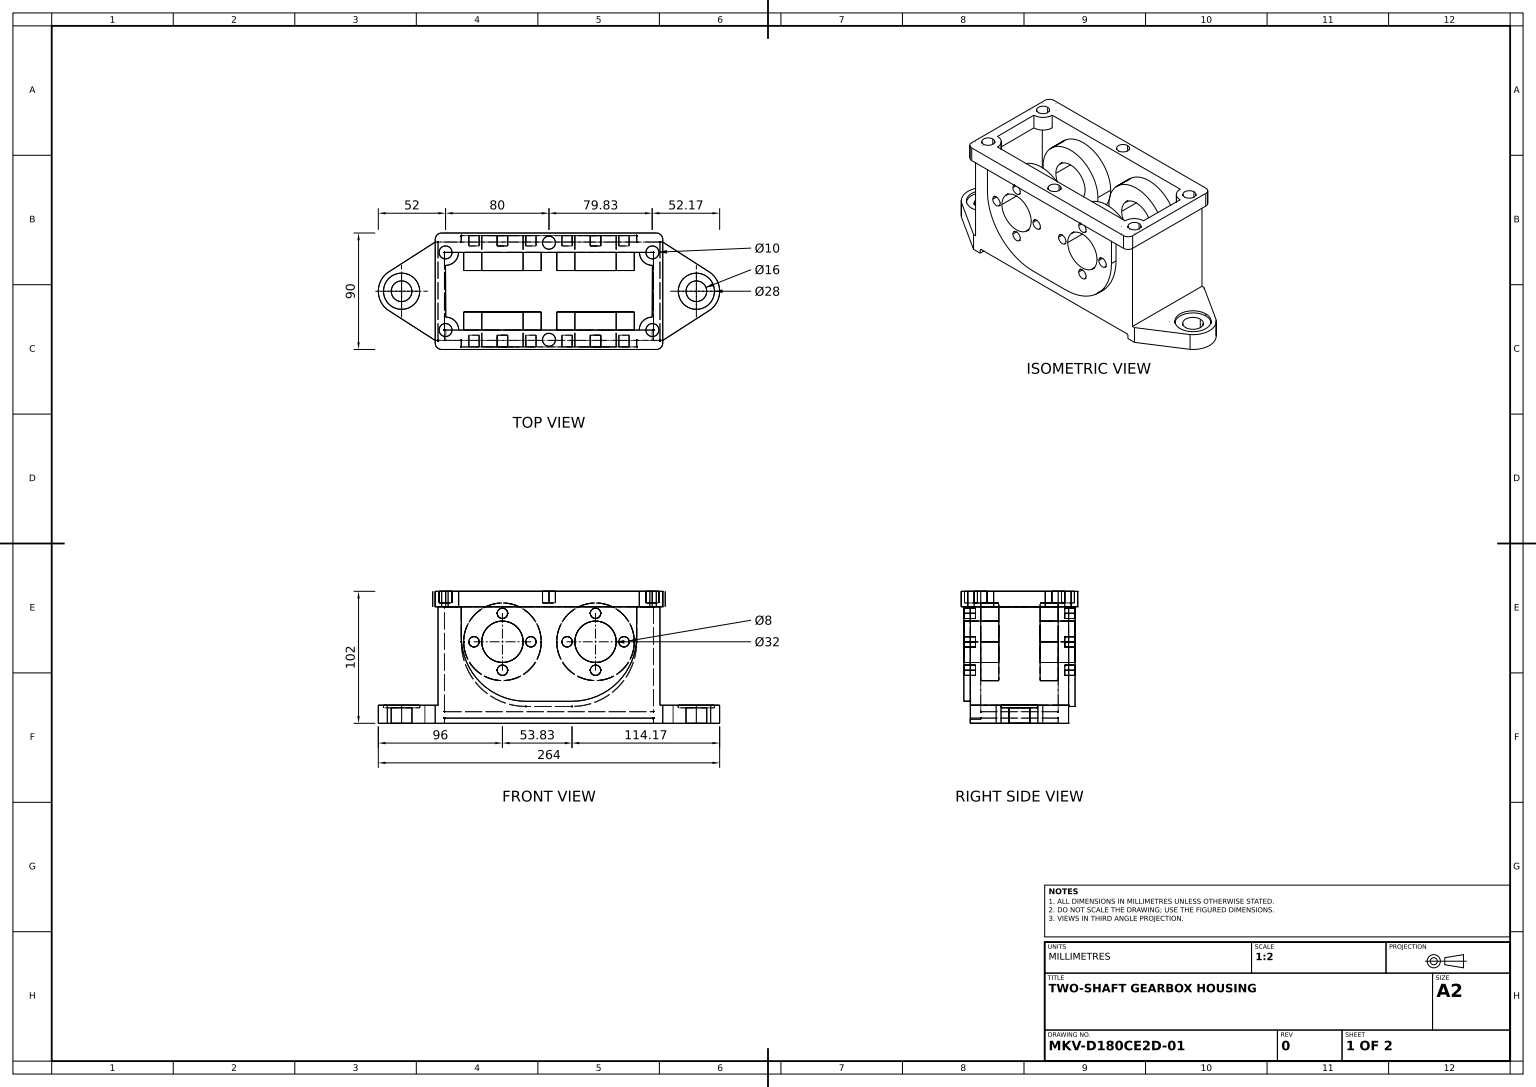
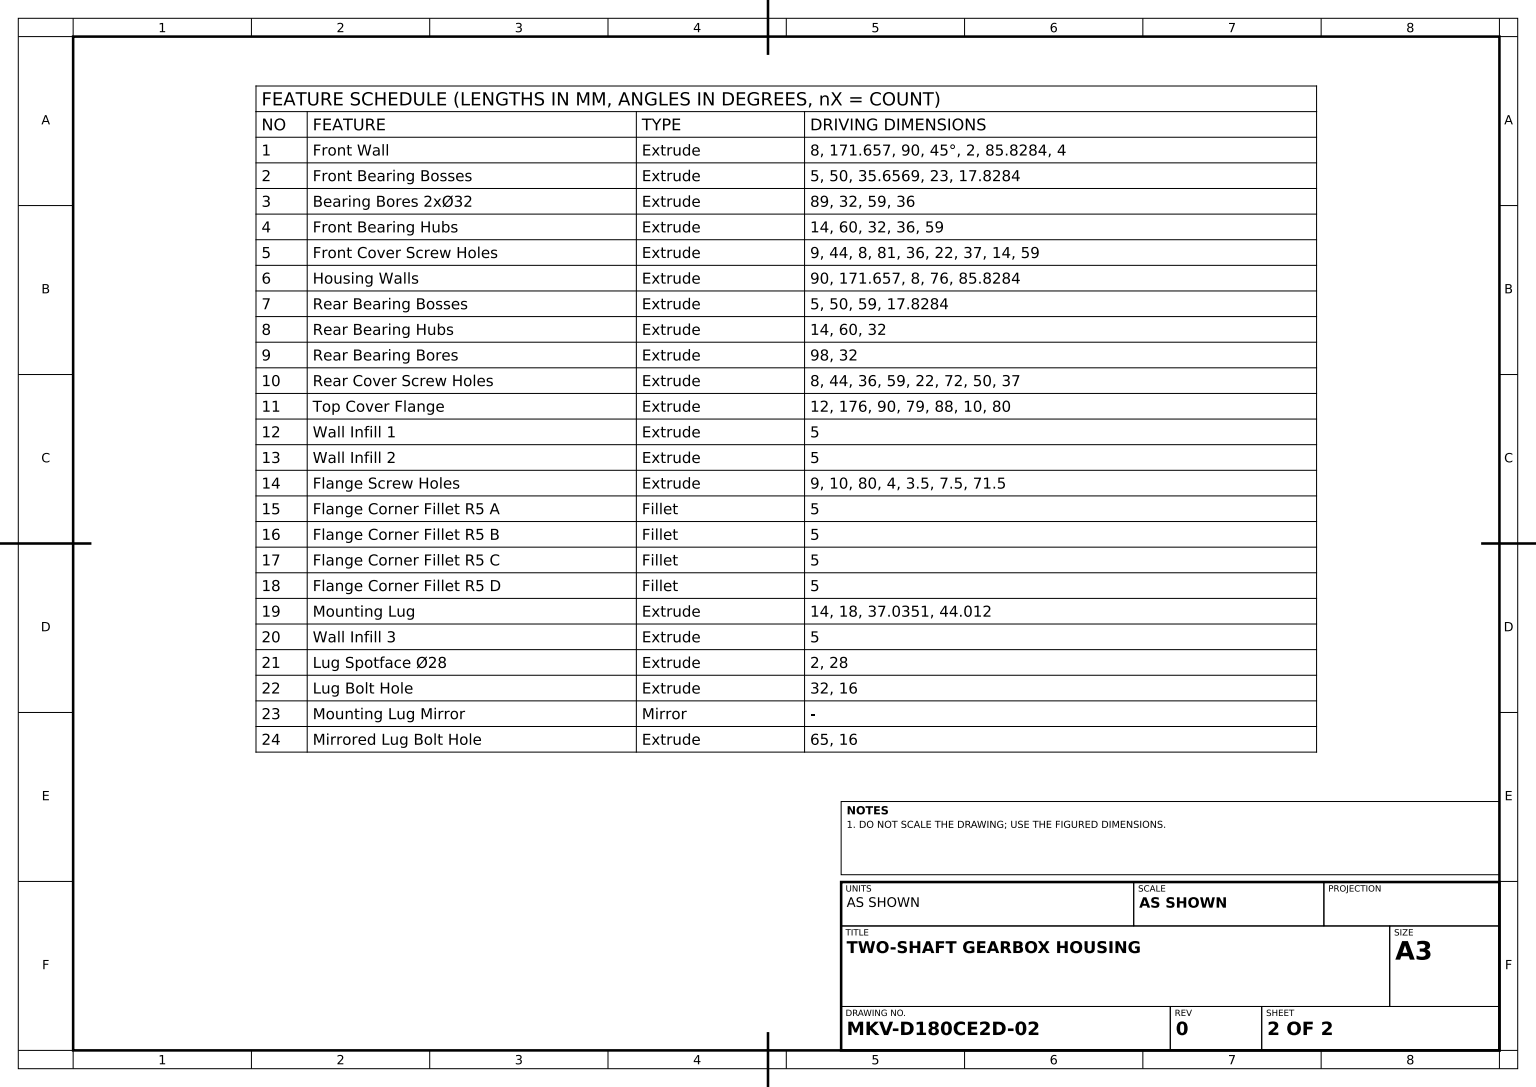
solid
v1 (-80,89,-59)
v2 (-80,98,-59)
e1 v1 v2 LINE
v3 (-80,98,-69)
e2 v2 v3 CIRCLE(AX(P(-80,98,-64),D(0,1,0),D(0,0,1)),5)
v4 (-80,89,-69)
e3 v4 v3 LINE
e4 v1 v4 CIRCLE(AX(P(-80,89,-64),D(0,1,0),D(0,0,1)),5)
face CYL(AX(P(-80,89,-64),D(0,1,0),D(0,0,1)),5) rev [e1 e2 -e3 -e4]
v5 (40,81,-77)
v6 (32,81,-77)
e5 v5 v6 CIRCLE(AX(P(36,81,-77),D(0,0,-1),D(1,0,0)),4)
v7 (32,81,-69)
e6 v7 v6 LINE
v8 (40,81,-69)
e7 v8 v7 CIRCLE(AX(P(36,81,-69),D(0,0,-1),D(1,0,0)),4)
e8 v8 v5 LINE
face CYL(AX(P(36,81,-69),D(0,0,-1),D(-1,0,0)),4) rev [e5 -e6 -e7 e8]
v9 (-69.828427,98,-4)
v10 (-79.828427,98,-14)
e9 v9 v10 CIRCLE(AX(P(-79.828427,98,-4),D(0,1,0),D(0,0,1)),10)
v11 (-69.828427,86,-4)
e10 v9 v11 LINE
v12 (-79.828427,86,-14)
e11 v11 v12 CIRCLE(AX(P(-79.828427,86,-4),D(0,1,0),D(0,0,1)),10)
e12 v10 v12 LINE
face CYL(AX(P(-79.828427,98,-4),D(0,-1,0),D(0,0,-1)),10) [-e9 e10 e11 -e12]
v13 (80,98,-59)
v14 (80,98,-69)
e13 v13 v14 CIRCLE(AX(P(80,98,-64),D(0,1,0),D(0,0,1)),5)
e14 v14 v13 CIRCLE(AX(P(80,98,-64),D(0,1,0),D(0,0,1)),5)
v15 (80,98,1)
v16 (80,98,-9)
e15 v15 v16 CIRCLE(AX(P(80,98,-4),D(0,1,0),D(0,0,-1)),5)
e16 v16 v15 CIRCLE(AX(P(80,98,-4),D(0,1,0),D(0,0,-1)),5)
v17 (0,98,-66.5)
v18 (0,98,-76.5)
e17 v17 v18 CIRCLE(AX(P(0,98,-71.5),D(0,1,0),D(0,0,1)),5)
e18 v18 v17 CIRCLE(AX(P(0,98,-71.5),D(0,1,0),D(0,0,1)),5)
v19 (83,98,-79)
v20 (-83,98,-79)
e19 v19 v20 LINE
v21 (-88,98,-74)
e20 v20 v21 CIRCLE(AX(P(-83,98,-74),D(0,1,0),D(0,0,1)),5)
v22 (-88,98,6)
e21 v21 v22 LINE
v23 (-83,98,11)
e22 v22 v23 CIRCLE(AX(P(-83,98,6),D(0,1,0),D(0,0,1)),5)
v24 (83,98,11)
e23 v23 v24 LINE
v25 (88,98,6)
e24 v24 v25 CIRCLE(AX(P(83,98,6),D(0,1,0),D(0,0,1)),5)
v26 (88,98,-74)
e25 v25 v26 LINE
e26 v26 v19 CIRCLE(AX(P(83,98,-74),D(0,1,0),D(0,0,1)),5)
e27 v3 v2 CIRCLE(AX(P(-80,98,-64),D(0,1,0),D(0,0,1)),5)
v27 (0,98,-1.5)
v28 (0,98,8.5)
e28 v27 v28 CIRCLE(AX(P(0,98,3.5),D(0,1,0),D(0,0,-1)),5)
e29 v28 v27 CIRCLE(AX(P(0,98,3.5),D(0,1,0),D(0,0,-1)),5)
v29 (-80,98,1)
v30 (-80,98,-9)
e30 v29 v30 CIRCLE(AX(P(-80,98,-4),D(0,1,0),D(0,0,-1)),5)
e31 v30 v29 CIRCLE(AX(P(-80,98,-4),D(0,1,0),D(0,0,-1)),5)
v31 (69.828427,98,-4)
v32 (79.828427,98,-14)
e32 v31 v32 CIRCLE(AX(P(79.828427,98,-4),D(0,-1,0),D(0,0,1)),10)
e33 v31 v9 LINE
v33 (-80,98,-54)
e34 v10 v33 LINE
v34 (-70,98,-64)
e35 v33 v34 CIRCLE(AX(P(-80,98,-64),D(0,1,0),D(0,0,1)),10)
v35 (70,98,-64)
e36 v34 v35 LINE
v36 (80,98,-54)
e37 v36 v35 CIRCLE(AX(P(80,98,-64),D(0,-1,0),D(0,0,1)),10)
e38 v36 v32 LINE
face PLANE(AX(P(0,98,0),D(0,1,0),D(0,0,1))) [-e13 -e14] [-e15 -e16] [-e17 -e18] [e19 e20 e21 e22 e23 e24 e25 e26] [-e27 -e2] [-e28 -e29] [-e30 -e31] [-e32 e33 e9 e34 e35 e36 -e37 e38]
v37 (70,86,-64)
e39 v35 v37 LINE
v38 (80,86,-54)
e40 v38 v37 CIRCLE(AX(P(80,86,-64),D(0,-1,0),D(0,0,1)),10)
e41 v36 v38 LINE
face CYL(AX(P(80,98,-64),D(0,-1,0),D(0,0,-1)),10) [e39 -e40 -e41 e37]
v39 (80,89,1)
e42 v39 v15 LINE
v40 (80,89,-9)
e43 v40 v16 LINE
e44 v39 v40 CIRCLE(AX(P(80,89,-4),D(0,1,0),D(0,0,-1)),5)
face CYL(AX(P(80,89,-4),D(0,1,0),D(0,0,1)),5) rev [e42 e15 -e43 -e44]
v41 (67.828427,59,-72)
v42 (17.828427,9,-72)
e45 v41 v42 CIRCLE(AX(P(17.828427,59,-72),D(0,0,-1),D(-1,0,0)),50)
v43 (17.828427,9,-77)
e46 v43 v42 LINE
v44 (67.828427,59,-77)
e47 v44 v43 CIRCLE(AX(P(17.828427,59,-77),D(0,0,-1),D(-1,0,0)),50)
e48 v44 v41 LINE
face CYL(AX(P(17.828427,59,-77),D(0,0,1),D(1,0,0)),50) [e45 -e46 -e47 e48]
v45 (-40,81,-69)
v46 (-40,81,-77)
e49 v45 v46 LINE
v47 (-32,81,-69)
e50 v47 v45 CIRCLE(AX(P(-36,81,-69),D(0,0,-1),D(-1,0,0)),4)
v48 (-32,81,-77)
e51 v47 v48 LINE
e52 v48 v46 CIRCLE(AX(P(-36,81,-77),D(0,0,-1),D(-1,0,0)),4)
face CYL(AX(P(-36,81,-69),D(0,0,-1),D(-1,0,0)),4) rev [-e49 -e50 e51 e52]
v49 (-80.828427,5,-64)
v50 (-80.828427,86,-64)
e53 v49 v50 LINE
v51 (80.828427,5,-64)
e54 v49 v51 LINE
v52 (80.828427,86,-64)
e55 v52 v51 LINE
e56 v37 v52 LINE
v53 (-70,86,-64)
e57 v34 v53 LINE
e58 v50 v53 LINE
v54 (66,59,-64)
v55 (6,59,-64)
e59 v54 v55 CIRCLE(AX(P(36,59,-64),D(0,0,1),D(1,0,0)),30)
e60 v55 v54 CIRCLE(AX(P(36,59,-64),D(0,0,1),D(1,0,0)),30)
v56 (-66,59,-64)
v57 (-6,59,-64)
e61 v56 v57 CIRCLE(AX(P(-36,59,-64),D(0,0,1),D(1,0,0)),30)
e62 v57 v56 CIRCLE(AX(P(-36,59,-64),D(0,0,1),D(1,0,0)),30)
face PLANE(AX(P(0,98,-64),D(0,0,-1),D(-1,0,0))) rev [-e53 e54 -e55 -e56 -e39 -e36 e57 -e58] [-e59 -e60] [-e61 -e62]
v58 (-17.828427,13,4)
v59 (17.828427,13,4)
e63 v58 v59 LINE
v60 (-67.828427,63,4)
e64 v60 v58 CIRCLE(AX(P(-17.828427,63,4),D(0,0,1),D(1,0,0)),50)
v61 (-67.828427,86,4)
e65 v61 v60 LINE
v62 (-85.828427,86,4)
e66 v61 v62 LINE
v63 (-85.828427,10,4)
e67 v62 v63 LINE
v64 (-88,10,4)
e68 v64 v63 LINE
v65 (-88,-4,4)
e69 v64 v65 LINE
v66 (-80.828427,-4,4)
e70 v65 v66 LINE
v67 (-80.828427,-1,4)
e71 v66 v67 LINE
v68 (-79.828427,0,4)
e72 v67 v68 LINE
v69 (79.828427,0,4)
e73 v68 v69 LINE
v70 (80.828427,-1,4)
e74 v69 v70 LINE
v71 (80.828427,-4,4)
e75 v70 v71 LINE
v72 (88,-4,4)
e76 v71 v72 LINE
v73 (88,10,4)
e77 v73 v72 LINE
v74 (85.828427,10,4)
e78 v73 v74 LINE
v75 (85.828427,86,4)
e79 v74 v75 LINE
v76 (67.828427,86,4)
e80 v75 v76 LINE
v77 (67.828427,63,4)
e81 v77 v76 LINE
e82 v59 v77 CIRCLE(AX(P(17.828427,63,4),D(0,0,1),D(1,0,0)),50)
face PLANE(AX(P(0,0,4),D(0,0,-1),D(-1,0,0))) rev [-e63 -e64 -e65 e66 e67 -e68 e69 e70 e71 e72 e73 e74 e75 e76 -e77 e78 e79 e80 -e81 -e82]
v78 (-40,37,-69)
v79 (-32,37,-69)
e83 v78 v79 CIRCLE(AX(P(-36,37,-69),D(0,0,-1),D(-1,0,0)),4)
e84 v79 v78 CIRCLE(AX(P(-36,37,-69),D(0,0,-1),D(-1,0,0)),4)
face PLANE(AX(P(-36,37,-69),D(0,0,-1),D(-1,0,0))) [e83 e84]
v80 (114,8,-42)
v81 (114,8,-26)
e85 v80 v81 CIRCLE(AX(P(114,8,-34),D(0,1,0),D(0,0,1)),8)
e86 v81 v80 CIRCLE(AX(P(114,8,-34),D(0,1,0),D(0,0,1)),8)
v82 (114,8,-20)
v83 (114,8,-48)
e87 v82 v83 CIRCLE(AX(P(114,8,-34),D(0,1,0),D(0,0,1)),14)
e88 v83 v82 CIRCLE(AX(P(114,8,-34),D(0,1,0),D(0,0,1)),14)
face PLANE(AX(P(114,8,-34),D(0,1,0),D(0,0,1))) [-e85 -e86] [e87 e88]
v84 (-32,37,0)
v85 (-40,37,0)
e89 v84 v85 CIRCLE(AX(P(-36,37,0),D(0,0,1),D(1,0,0)),4)
e90 v85 v84 CIRCLE(AX(P(-36,37,0),D(0,0,1),D(1,0,0)),4)
face PLANE(AX(P(-36,37,0),D(0,0,1),D(1,0,0))) [e89 e90]
v86 (-66,59,-18)
v87 (-6,59,-18)
e91 v86 v87 CIRCLE(AX(P(-36,59,-18),D(0,0,-1),D(-1,0,0)),30)
v88 (-66,59,-4)
e92 v86 v88 LINE
v89 (-6,59,-4)
e93 v88 v89 CIRCLE(AX(P(-36,59,-4),D(0,0,-1),D(-1,0,0)),30)
e94 v87 v89 LINE
face CYL(AX(P(-36,59,-18),D(0,0,1),D(1,0,0)),30) [-e91 e92 e93 -e94]
v90 (-88,86,-74)
e95 v21 v90 LINE
v91 (-88,86,6)
e96 v90 v91 LINE
e97 v91 v22 LINE
face PLANE(AX(P(-88,98,0),D(1,0,0),D(0,0,-1))) rev [e95 e96 e97 -e21]
v92 (-32,37,9)
e98 v84 v92 LINE
v93 (-40,37,9)
e99 v92 v93 CIRCLE(AX(P(-36,37,9),D(0,0,1),D(1,0,0)),4)
e100 v85 v93 LINE
face CYL(AX(P(-36,37,0),D(0,0,1),D(1,0,0)),4) rev [e98 e99 -e100 -e89]
v94 (79.828427,86,-14)
e101 v38 v94 LINE
e102 v32 v94 LINE
face PLANE(AX(P(79.766909,98,0.342146),D(0.999990801,0,0.004289282),D(0.004289282,0,-0.999990801))) rev [-e38 e41 e101 -e102]
v95 (-83,86,11)
v96 (83,86,11)
e103 v95 v96 LINE
e104 v96 v24 LINE
e105 v23 v95 LINE
face PLANE(AX(P(0,98,11),D(0,0,-1),D(-1,0,0))) rev [e103 e104 -e23 e105]
v97 (-40,81,9)
v98 (-32,81,9)
e106 v97 v98 CIRCLE(AX(P(-36,81,9),D(0,0,1),D(1,0,0)),4)
v99 (-32,81,0)
e107 v99 v98 LINE
v100 (-40,81,0)
e108 v100 v99 CIRCLE(AX(P(-36,81,0),D(0,0,1),D(1,0,0)),4)
e109 v100 v97 LINE
face CYL(AX(P(-36,81,0),D(0,0,1),D(1,0,0)),4) rev [e106 -e107 -e108 e109]
v101 (-52,59,-50)
v102 (-52,59,-77)
e110 v101 v102 LINE
v103 (-20,59,-50)
e111 v101 v103 CIRCLE(AX(P(-36,59,-50),D(0,0,1),D(1,0,0)),16)
v104 (-20,59,-77)
e112 v103 v104 LINE
e113 v104 v102 CIRCLE(AX(P(-36,59,-77),D(0,0,-1),D(-1,0,0)),16)
face CYL(AX(P(-36,59,-50),D(0,0,-1),D(-1,0,0)),16) rev [-e110 e111 e112 e113]
v105 (88,10,-72)
v106 (125.035091,10,-48.220646)
e114 v105 v106 LINE
v107 (125.035091,-4,-48.220646)
e115 v106 v107 LINE
v108 (88,-4,-72)
e116 v108 v107 LINE
e117 v105 v108 LINE
face PLANE(AX(P(88,10,-72),D(0.540292585,0,-0.841477227),D(-0.841477227,0,-0.540292585))) [e114 e115 -e116 -e117]
v109 (20,59,-18)
v110 (52,59,-18)
e118 v109 v110 CIRCLE(AX(P(36,59,-18),D(0,0,-1),D(1,0,0)),16)
e119 v110 v109 CIRCLE(AX(P(36,59,-18),D(0,0,-1),D(1,0,0)),16)
v111 (6,59,-18)
v112 (66,59,-18)
e120 v111 v112 CIRCLE(AX(P(36,59,-18),D(0,0,-1),D(1,0,0)),30)
e121 v112 v111 CIRCLE(AX(P(36,59,-18),D(0,0,-1),D(1,0,0)),30)
face PLANE(AX(P(36,59,-18),D(0,0,1),D(1,0,0))) rev [-e118 -e119] [e120 e121]
v113 (20,59,-77)
v114 (52,59,-77)
e122 v113 v114 CIRCLE(AX(P(36,59,-77),D(0,0,-1),D(-1,0,0)),16)
v115 (52,59,-50)
e123 v115 v114 LINE
v116 (20,59,-50)
e124 v115 v116 CIRCLE(AX(P(36,59,-50),D(0,0,1),D(1,0,0)),16)
e125 v116 v113 LINE
face CYL(AX(P(36,59,-50),D(0,0,-1),D(-1,0,0)),16) rev [e122 -e123 e124 e125]
v117 (-114,-4,-26)
v118 (-114,8,-26)
e126 v117 v118 LINE
v119 (-114,8,-42)
e127 v118 v119 CIRCLE(AX(P(-114,8,-34),D(0,1,0),D(0,0,1)),8)
v120 (-114,-4,-42)
e128 v120 v119 LINE
e129 v117 v120 CIRCLE(AX(P(-114,-4,-34),D(0,1,0),D(0,0,1)),8)
face CYL(AX(P(-114,-57,-34),D(0,1,0),D(0,0,1)),8) rev [e126 e127 -e128 -e129]
v121 (80.828427,0,-64)
v122 (80.828427,0,-4)
e130 v121 v122 LINE
v123 (80.828427,-4,-64)
e131 v121 v123 LINE
e132 v71 v123 LINE
v124 (80.828427,-1,-4)
e133 v70 v124 LINE
e134 v122 v124 LINE
face PLANE(AX(P(80.828427,0,0),D(1,0,0),D(0,0,-1))) rev [-e130 e131 -e132 -e75 e133 -e134]
v125 (-80.828427,5,-4)
v126 (-80.828427,86,-4)
e135 v125 v126 LINE
e136 v125 v49 LINE
e137 v50 v126 LINE
face PLANE(AX(P(-80.828427,0,0),D(-1,0,0),D(0,0,1))) rev [-e135 e136 e53 e137]
v127 (20,59,9)
e138 v109 v127 LINE
v128 (52,59,9)
e139 v127 v128 CIRCLE(AX(P(36,59,9),D(0,0,1),D(-1,0,0)),16)
e140 v110 v128 LINE
face CYL(AX(P(36,59,-80),D(0,0,1),D(1,0,0)),16) rev [e138 e139 -e140 e119]
v129 (62,59,-69)
v130 (54,59,-69)
e141 v129 v130 CIRCLE(AX(P(58,59,-69),D(0,0,-1),D(1,0,0)),4)
e142 v130 v129 CIRCLE(AX(P(58,59,-69),D(0,0,-1),D(1,0,0)),4)
face PLANE(AX(P(58,59,-69),D(0,0,1),D(1,0,0))) rev [e141 e142]
e143 v40 v39 CIRCLE(AX(P(80,89,-4),D(0,1,0),D(0,0,-1)),5)
face CYL(AX(P(80,89,-4),D(0,1,0),D(0,0,1)),5) rev [e43 e16 -e42 -e143]
v131 (62,59,-77)
v132 (54,59,-77)
e144 v131 v132 CIRCLE(AX(P(58,59,-77),D(0,0,-1),D(1,0,0)),4)
e145 v130 v132 LINE
e146 v129 v131 LINE
face CYL(AX(P(58,59,-69),D(0,0,-1),D(-1,0,0)),4) rev [e144 -e145 -e141 e146]
v133 (67.828427,86,9)
e147 v133 v76 LINE
v134 (67.828427,63,9)
e148 v134 v133 LINE
e149 v134 v77 LINE
face PLANE(AX(P(67.828427,63,9),D(-1,0,0),D(0,0,1))) rev [e81 -e147 -e148 e149]
v135 (-88,-4,-72)
e150 v108 v135 LINE
v136 (-88,10,-72)
e151 v136 v135 LINE
v137 (-85.828427,10,-72)
e152 v137 v136 LINE
v138 (-85.828427,86,-72)
e153 v137 v138 LINE
v139 (-67.828427,86,-72)
e154 v139 v138 LINE
v140 (-67.828427,59,-72)
e155 v140 v139 LINE
v141 (-17.828427,9,-72)
e156 v141 v140 CIRCLE(AX(P(-17.828427,59,-72),D(0,0,-1),D(-1,0,0)),50)
e157 v42 v141 LINE
v142 (67.828427,86,-72)
e158 v142 v41 LINE
v143 (85.828427,86,-72)
e159 v143 v142 LINE
v144 (85.828427,10,-72)
e160 v144 v143 LINE
e161 v144 v105 LINE
face PLANE(AX(P(85.828427,-4,-72),D(0,0,-1),D(-1,0,0))) [e117 e150 -e151 -e152 e153 -e154 -e155 -e156 -e157 -e45 -e158 -e159 -e160 e161]
v145 (-54,59,0)
v146 (-62,59,0)
e162 v145 v146 CIRCLE(AX(P(-58,59,0),D(0,0,1),D(1,0,0)),4)
v147 (-54,59,9)
e163 v145 v147 LINE
v148 (-62,59,9)
e164 v147 v148 CIRCLE(AX(P(-58,59,9),D(0,0,1),D(1,0,0)),4)
e165 v146 v148 LINE
face CYL(AX(P(-58,59,0),D(0,0,1),D(1,0,0)),4) rev [-e162 e163 e164 -e165]
v149 (-114,8,-48)
v150 (-114,10,-48)
e166 v149 v150 LINE
v151 (-114,10,-20)
e167 v151 v150 CIRCLE(AX(P(-114,10,-34),D(0,-1,0),D(0,0,1)),14)
v152 (-114,8,-20)
e168 v152 v151 LINE
e169 v152 v149 CIRCLE(AX(P(-114,8,-34),D(0,-1,0),D(0,0,1)),14)
face CYL(AX(P(-114,8,-34),D(0,1,0),D(0,0,1)),14) rev [e166 -e167 -e168 e169]
v153 (-18,59,-77)
v154 (-10,59,-77)
e170 v153 v154 CIRCLE(AX(P(-14,59,-77),D(0,0,-1),D(-1,0,0)),4)
v155 (-10,59,-69)
e171 v155 v154 LINE
v156 (-18,59,-69)
e172 v156 v155 CIRCLE(AX(P(-14,59,-69),D(0,0,-1),D(-1,0,0)),4)
e173 v156 v153 LINE
face CYL(AX(P(-14,59,-69),D(0,0,-1),D(-1,0,0)),4) rev [e170 -e171 -e172 e173]
e174 v150 v151 CIRCLE(AX(P(-114,10,-34),D(0,-1,0),D(0,0,1)),14)
e175 v149 v152 CIRCLE(AX(P(-114,8,-34),D(0,-1,0),D(0,0,1)),14)
face CYL(AX(P(-114,8,-34),D(0,1,0),D(0,0,1)),14) rev [e168 -e174 -e166 e175]
v157 (0,89,8.5)
v158 (0,89,-1.5)
e176 v157 v158 CIRCLE(AX(P(0,89,3.5),D(0,1,0),D(0,0,-1)),5)
e177 v158 v157 CIRCLE(AX(P(0,89,3.5),D(0,1,0),D(0,0,-1)),5)
face PLANE(AX(P(0,89,3.5),D(0,-1,0),D(0,0,-1))) rev [e176 e177]
v159 (69.828427,86,-4)
e178 v31 v159 LINE
v160 (80.828427,86,-4)
e179 v160 v159 LINE
v161 (80.828427,5,-4)
e180 v160 v161 LINE
e181 v125 v161 LINE
e182 v126 v11 LINE
e183 v89 v88 CIRCLE(AX(P(-36,59,-4),D(0,0,-1),D(-1,0,0)),30)
v162 (66,59,-4)
v163 (6,59,-4)
e184 v162 v163 CIRCLE(AX(P(36,59,-4),D(0,0,-1),D(1,0,0)),30)
e185 v163 v162 CIRCLE(AX(P(36,59,-4),D(0,0,-1),D(1,0,0)),30)
face PLANE(AX(P(0,0,-4),D(0,0,-1),D(-1,0,0))) [e178 -e179 e180 -e181 e135 e182 -e10 -e33] [-e183 -e93] [-e184 -e185]
e186 v103 v101 CIRCLE(AX(P(-36,59,-50),D(0,0,1),D(1,0,0)),16)
e187 v102 v104 CIRCLE(AX(P(-36,59,-77),D(0,0,-1),D(-1,0,0)),16)
face CYL(AX(P(-36,59,-50),D(0,0,-1),D(-1,0,0)),16) rev [-e112 e186 e110 e187]
e188 v119 v118 CIRCLE(AX(P(-114,8,-34),D(0,1,0),D(0,0,1)),8)
face PLANE(AX(P(-114,8,-34),D(0,1,0),D(0,0,1))) [-e175 -e169] [-e127 -e188]
v164 (-10,59,0)
v165 (-18,59,0)
e189 v164 v165 CIRCLE(AX(P(-14,59,0),D(0,0,1),D(1,0,0)),4)
e190 v165 v164 CIRCLE(AX(P(-14,59,0),D(0,0,1),D(1,0,0)),4)
face PLANE(AX(P(-14,59,0),D(0,0,1),D(1,0,0))) [e189 e190]
v166 (125.035091,-4,-19.779354)
e191 v166 v72 LINE
v167 (-80.828427,-4,-64)
e192 v167 v123 LINE
e193 v167 v66 LINE
v168 (-125.035091,-4,-19.779354)
e194 v168 v65 LINE
v169 (-125.035091,-4,-48.220646)
e195 v169 v168 CIRCLE(AX(P(-114,-4,-34),D(0,1,0),D(0,0,-1)),18)
e196 v135 v169 LINE
e197 v107 v166 CIRCLE(AX(P(114,-4,-34),D(0,-1,0),D(0,0,-1)),18)
e198 v120 v117 CIRCLE(AX(P(-114,-4,-34),D(0,1,0),D(0,0,1)),8)
v170 (114,-4,-42)
v171 (114,-4,-26)
e199 v170 v171 CIRCLE(AX(P(114,-4,-34),D(0,1,0),D(0,0,1)),8)
e200 v171 v170 CIRCLE(AX(P(114,-4,-34),D(0,1,0),D(0,0,1)),8)
face PLANE(AX(P(-83.828427,-4,4),D(0,1,0),D(0,0,1))) rev [e191 -e76 e132 -e192 e193 -e70 -e194 -e195 -e196 -e150 e116 e197] [e129 e198] [e199 e200]
v172 (-80.828427,0,-4)
v173 (-79.828427,0,-4)
e201 v172 v173 LINE
v174 (-80.828427,-1,-4)
e202 v174 v173 LINE
e203 v174 v172 LINE
face PLANE(AX(P(0,0,-4),D(0,0,-1),D(-1,0,0))) [e201 -e202 e203]
v175 (-80,86,-54)
e204 v33 v175 LINE
e205 v175 v53 CIRCLE(AX(P(-80,86,-64),D(0,1,0),D(0,0,1)),10)
face CYL(AX(P(-80,98,-64),D(0,-1,0),D(0,0,-1)),10) [-e35 e204 e205 -e57]
v176 (-80,89,1)
e206 v176 v29 LINE
v177 (-80,89,-9)
e207 v177 v176 CIRCLE(AX(P(-80,89,-4),D(0,1,0),D(0,0,-1)),5)
e208 v177 v30 LINE
face CYL(AX(P(-80,89,-4),D(0,1,0),D(0,0,1)),5) rev [e31 -e206 -e207 e208]
v178 (80,89,-69)
e209 v178 v14 LINE
v179 (80,89,-59)
e210 v179 v178 CIRCLE(AX(P(80,89,-64),D(0,1,0),D(0,0,1)),5)
e211 v179 v13 LINE
face CYL(AX(P(80,89,-64),D(0,1,0),D(0,0,1)),5) rev [e13 -e209 -e210 e211]
e212 v74 v144 LINE
e213 v75 v143 LINE
face PLANE(AX(P(85.828427,-4,4),D(-1,0,0),D(0,0,1))) rev [-e79 e212 e160 -e213]
v180 (-83,86,-79)
e214 v90 v180 CIRCLE(AX(P(-83,86,-74),D(0,-1,0),D(0,0,1)),5)
e215 v180 v20 LINE
face CYL(AX(P(-83,98,-74),D(0,-1,0),D(0,0,-1)),5) [-e214 -e95 -e20 -e215]
v181 (18,59,-69)
v182 (10,59,-69)
e216 v181 v182 CIRCLE(AX(P(14,59,-69),D(0,0,-1),D(1,0,0)),4)
e217 v182 v181 CIRCLE(AX(P(14,59,-69),D(0,0,-1),D(1,0,0)),4)
face PLANE(AX(P(14,59,-69),D(0,0,1),D(1,0,0))) rev [e216 e217]
e218 v63 v137 LINE
e219 v62 v138 LINE
face PLANE(AX(P(-85.828427,-4,4),D(1,0,0),D(0,0,-1))) rev [-e153 -e218 -e67 e219]
e220 v68 v173 LINE
e221 v174 v67 LINE
face PLANE(AX(P(-79.828427,0,4),D(-0.707106781,0.707106781,0),D(-0.707106781,-0.707106781,0))) rev [e202 -e220 -e72 -e221]
v183 (17.828427,13,9)
e222 v183 v134 CIRCLE(AX(P(17.828427,63,9),D(0,0,1),D(1,0,0)),50)
e223 v183 v59 LINE
face CYL(AX(P(17.828427,63,9),D(0,0,-1),D(-1,0,0)),50) [-e149 -e222 e223 e82]
v184 (114,10,-20)
v185 (114,10,-48)
e224 v184 v185 CIRCLE(AX(P(114,10,-34),D(0,1,0),D(0,0,1)),14)
e225 v185 v184 CIRCLE(AX(P(114,10,-34),D(0,1,0),D(0,0,1)),14)
v186 (125.035091,10,-19.779354)
e226 v186 v73 LINE
e227 v106 v186 CIRCLE(AX(P(114,10,-34),D(0,-1,0),D(0,0,-1)),18)
face PLANE(AX(P(114,10,-34),D(0,-1,0),D(0,0,-1))) rev [-e224 -e225] [-e78 -e226 -e227 -e114 -e161 -e212]
v187 (-6,59,-50)
e228 v187 v57 LINE
v188 (-66,59,-50)
e229 v188 v56 LINE
e230 v187 v188 CIRCLE(AX(P(-36,59,-50),D(0,0,1),D(1,0,0)),30)
face CYL(AX(P(-36,59,-50),D(0,0,-1),D(-1,0,0)),30) [e228 e62 -e229 -e230]
e231 v95 v91 CIRCLE(AX(P(-83,86,6),D(0,-1,0),D(0,0,1)),5)
face CYL(AX(P(-83,98,6),D(0,-1,0),D(0,0,-1)),5) [-e97 -e231 -e105 -e22]
v189 (-17.828427,9,-77)
v190 (-67.828427,59,-77)
e232 v189 v190 CIRCLE(AX(P(-17.828427,59,-77),D(0,0,-1),D(-1,0,0)),50)
e233 v189 v141 LINE
e234 v190 v140 LINE
face CYL(AX(P(-17.828427,59,-77),D(0,0,1),D(1,0,0)),50) [-e232 e233 e156 -e234]
e235 v93 v92 CIRCLE(AX(P(-36,37,9),D(0,0,1),D(1,0,0)),4)
v191 (40,37,9)
v192 (32,37,9)
e236 v191 v192 CIRCLE(AX(P(36,37,9),D(0,0,1),D(-1,0,0)),4)
e237 v192 v191 CIRCLE(AX(P(36,37,9),D(0,0,1),D(-1,0,0)),4)
v193 (40,81,9)
v194 (32,81,9)
e238 v193 v194 CIRCLE(AX(P(36,81,9),D(0,0,1),D(-1,0,0)),4)
e239 v194 v193 CIRCLE(AX(P(36,81,9),D(0,0,1),D(-1,0,0)),4)
v195 (-18,59,9)
v196 (-10,59,9)
e240 v195 v196 CIRCLE(AX(P(-14,59,9),D(0,0,1),D(1,0,0)),4)
e241 v196 v195 CIRCLE(AX(P(-14,59,9),D(0,0,1),D(1,0,0)),4)
v197 (62,59,9)
v198 (54,59,9)
e242 v197 v198 CIRCLE(AX(P(58,59,9),D(0,0,1),D(-1,0,0)),4)
e243 v198 v197 CIRCLE(AX(P(58,59,9),D(0,0,1),D(-1,0,0)),4)
e244 v148 v147 CIRCLE(AX(P(-58,59,9),D(0,0,1),D(1,0,0)),4)
e245 v128 v127 CIRCLE(AX(P(36,59,9),D(0,0,1),D(-1,0,0)),16)
v199 (10,59,9)
v200 (18,59,9)
e246 v199 v200 CIRCLE(AX(P(14,59,9),D(0,0,1),D(-1,0,0)),4)
e247 v200 v199 CIRCLE(AX(P(14,59,9),D(0,0,1),D(-1,0,0)),4)
e248 v98 v97 CIRCLE(AX(P(-36,81,9),D(0,0,1),D(1,0,0)),4)
v201 (-52,59,9)
v202 (-20,59,9)
e249 v201 v202 CIRCLE(AX(P(-36,59,9),D(0,0,1),D(1,0,0)),16)
e250 v202 v201 CIRCLE(AX(P(-36,59,9),D(0,0,1),D(1,0,0)),16)
v203 (-67.828427,86,9)
v204 (-67.828427,63,9)
e251 v203 v204 LINE
v205 (-17.828427,13,9)
e252 v204 v205 CIRCLE(AX(P(-17.828427,63,9),D(0,0,1),D(1,0,0)),50)
e253 v205 v183 LINE
e254 v133 v203 LINE
face PLANE(AX(P(-17.828427,63,9),D(0,0,1),D(1,0,0))) [-e235 -e99] [-e236 -e237] [-e238 -e239] [-e240 -e241] [-e242 -e243] [-e244 -e164] [-e245 -e139] [-e246 -e247] [-e106 -e248] [-e249 -e250] [e251 e252 e253 e222 e148 e254]
e255 v158 v27 LINE
e256 v157 v28 LINE
face CYL(AX(P(0,89,3.5),D(0,1,0),D(0,0,1)),5) rev [e29 -e255 -e176 e256]
e257 v12 v175 LINE
face PLANE(AX(P(-79.766909,98,0.342146),D(-0.999990801,0,0.004289282),D(0.004289282,0,0.999990801))) rev [-e204 -e34 e12 e257]
v206 (79.828427,0,-4)
e258 v69 v206 LINE
e259 v206 v124 LINE
face PLANE(AX(P(79.828427,0,4),D(0.707106781,0.707106781,0),D(-0.707106781,0.707106781,0))) rev [e258 e259 -e133 -e74]
v207 (-40,37,-77)
e260 v78 v207 LINE
v208 (-32,37,-77)
e261 v79 v208 LINE
e262 v208 v207 CIRCLE(AX(P(-36,37,-77),D(0,0,-1),D(-1,0,0)),4)
face CYL(AX(P(-36,37,-69),D(0,0,-1),D(-1,0,0)),4) rev [-e260 -e84 e261 e262]
e263 v188 v187 CIRCLE(AX(P(-36,59,-50),D(0,0,1),D(1,0,0)),30)
face PLANE(AX(P(-36,59,-50),D(0,0,1),D(1,0,0))) [e230 e263] [-e111 -e186]
e264 v206 v122 LINE
face PLANE(AX(P(0,0,-4),D(0,0,-1),D(-1,0,0))) [-e259 e264 e134]
e265 v99 v100 CIRCLE(AX(P(-36,81,0),D(0,0,1),D(1,0,0)),4)
face PLANE(AX(P(-36,81,0),D(0,0,1),D(1,0,0))) [e108 e265]
face CYL(AX(P(36,59,-80),D(0,0,1),D(1,0,0)),16) rev [e245 -e138 e118 e140]
v209 (-80.828427,0,-64)
e266 v172 v209 LINE
e267 v209 v121 LINE
face PLANE(AX(P(0,0,4),D(0,1,0),D(0,0,1))) rev [e220 -e201 e266 e267 e130 -e264 -e258 -e73]
e268 v51 v161 LINE
face PLANE(AX(P(0,5,0),D(0,1,0),D(0,0,1))) [e181 -e268 -e54 -e136]
v210 (-125.035091,10,-48.220646)
e269 v136 v210 LINE
v211 (-125.035091,10,-19.779354)
e270 v210 v211 CIRCLE(AX(P(-114,10,-34),D(0,1,0),D(0,0,-1)),18)
e271 v211 v64 LINE
face PLANE(AX(P(-114,10,-34),D(0,-1,0),D(0,0,-1))) rev [e174 e167] [e218 e152 e269 e270 e271 e68]
e272 v211 v168 LINE
e273 v210 v169 LINE
face CYL(AX(P(-114,10,-34),D(0,-1,0),D(0,0,-1)),18) [e195 -e272 -e270 e273]
v212 (-67.828427,86,-77)
e274 v212 v139 LINE
e275 v203 v61 LINE
v213 (67.828427,86,-77)
e276 v213 v142 LINE
e277 v212 v213 LINE
v214 (88,86,6)
e278 v214 v96 CIRCLE(AX(P(83,86,6),D(0,-1,0),D(0,0,1)),5)
v215 (83,86,-79)
e279 v215 v180 LINE
v216 (88,86,-74)
e280 v215 v216 CIRCLE(AX(P(83,86,-74),D(0,-1,0),D(0,0,1)),5)
e281 v214 v216 LINE
face PLANE(AX(P(0,86,0),D(0,1,0),D(0,0,1))) rev [e274 e154 -e219 -e66 -e275 -e254 e147 -e80 e213 e159 -e276 -e277] [e278 -e103 e231 -e96 e214 -e279 e280 -e281]
e282 v178 v179 CIRCLE(AX(P(80,89,-64),D(0,1,0),D(0,0,1)),5)
face PLANE(AX(P(80,89,-64),D(0,1,0),D(0,0,1))) [e282 e210]
face CYL(AX(P(-114,-57,-34),D(0,1,0),D(0,0,1)),8) rev [-e198 e128 e188 -e126]
e283 v204 v60 LINE
face PLANE(AX(P(-67.828427,86,9),D(1,0,0),D(0,1,0))) rev [e275 e65 -e283 -e251]
v217 (10,59,0)
e284 v217 v199 LINE
v218 (18,59,0)
e285 v218 v200 LINE
e286 v217 v218 CIRCLE(AX(P(14,59,0),D(0,0,1),D(-1,0,0)),4)
face CYL(AX(P(14,59,0),D(0,0,1),D(1,0,0)),4) rev [e284 e246 -e285 -e286]
e287 v186 v166 LINE
face PLANE(AX(P(88,10,4),D(0.540292585,0,0.841477227),D(0.841477227,0,-0.540292585))) [e226 e77 -e191 -e287]
e288 v216 v26 LINE
e289 v19 v215 LINE
face CYL(AX(P(83,98,-74),D(0,-1,0),D(0,0,-1)),5) [-e288 -e280 -e289 -e26]
v219 (54,59,0)
v220 (62,59,0)
e290 v219 v220 CIRCLE(AX(P(58,59,0),D(0,0,1),D(-1,0,0)),4)
e291 v219 v198 LINE
e292 v220 v197 LINE
face CYL(AX(P(58,59,0),D(0,0,1),D(1,0,0)),4) rev [-e290 e291 e243 -e292]
v221 (32,81,0)
e293 v221 v194 LINE
v222 (40,81,0)
e294 v222 v221 CIRCLE(AX(P(36,81,0),D(0,0,1),D(-1,0,0)),4)
e295 v222 v193 LINE
face CYL(AX(P(36,81,0),D(0,0,1),D(1,0,0)),4) rev [e238 -e293 -e294 e295]
e296 v82 v184 LINE
e297 v83 v185 LINE
face CYL(AX(P(114,8,-34),D(0,1,0),D(0,0,1)),14) rev [-e87 e296 e224 -e297]
face CYL(AX(P(0,89,3.5),D(0,1,0),D(0,0,1)),5) rev [e28 -e256 -e177 e255]
v223 (-52,59,-18)
e298 v223 v201 LINE
v224 (-20,59,-18)
e299 v224 v202 LINE
e300 v224 v223 CIRCLE(AX(P(-36,59,-18),D(0,0,-1),D(-1,0,0)),16)
face CYL(AX(P(-36,59,-80),D(0,0,1),D(1,0,0)),16) rev [e298 e249 -e299 e300]
e301 v223 v224 CIRCLE(AX(P(-36,59,-18),D(0,0,-1),D(-1,0,0)),16)
face CYL(AX(P(-36,59,-80),D(0,0,1),D(1,0,0)),16) rev [e299 e250 -e298 e301]
v225 (32,37,0)
e302 v225 v192 LINE
v226 (40,37,0)
e303 v226 v225 CIRCLE(AX(P(36,37,0),D(0,0,1),D(-1,0,0)),4)
e304 v226 v191 LINE
face CYL(AX(P(36,37,0),D(0,0,1),D(1,0,0)),4) rev [e236 -e302 -e303 e304]
v227 (40,37,-69)
v228 (32,37,-69)
e305 v227 v228 CIRCLE(AX(P(36,37,-69),D(0,0,-1),D(1,0,0)),4)
e306 v228 v227 CIRCLE(AX(P(36,37,-69),D(0,0,-1),D(1,0,0)),4)
face PLANE(AX(P(36,37,-69),D(0,0,1),D(1,0,0))) rev [e305 e306]
v229 (-54,59,-69)
v230 (-54,59,-77)
e307 v229 v230 LINE
v231 (-62,59,-69)
e308 v231 v229 CIRCLE(AX(P(-58,59,-69),D(0,0,-1),D(-1,0,0)),4)
v232 (-62,59,-77)
e309 v231 v232 LINE
e310 v232 v230 CIRCLE(AX(P(-58,59,-77),D(0,0,-1),D(-1,0,0)),4)
face CYL(AX(P(-58,59,-69),D(0,0,-1),D(-1,0,0)),4) rev [-e307 -e308 e309 e310]
e311 v114 v113 CIRCLE(AX(P(36,59,-77),D(0,0,-1),D(-1,0,0)),16)
e312 v116 v115 CIRCLE(AX(P(36,59,-50),D(0,0,1),D(1,0,0)),16)
face CYL(AX(P(36,59,-50),D(0,0,-1),D(-1,0,0)),16) rev [e311 -e125 e312 e123]
e313 v213 v44 LINE
face PLANE(AX(P(67.828427,86,-77),D(-1,0,0),D(0,0,1))) rev [e158 -e48 -e313 e276]
e314 v159 v94 CIRCLE(AX(P(79.828427,86,-4),D(0,-1,0),D(0,0,1)),10)
e315 v160 v52 LINE
face PLANE(AX(P(0,86,0),D(0,1,0),D(0,0,1))) rev [e179 e314 -e101 e40 e56 -e315]
e316 v87 v86 CIRCLE(AX(P(-36,59,-18),D(0,0,-1),D(-1,0,0)),30)
face PLANE(AX(P(-36,59,-18),D(0,0,-1),D(-1,0,0))) [-e300 -e301] [e91 e316]
face CYL(AX(P(79.828427,98,-4),D(0,-1,0),D(0,0,-1)),10) [-e314 -e178 e32 e102]
v233 (66,59,-50)
e317 v233 v54 LINE
v234 (6,59,-50)
e318 v234 v233 CIRCLE(AX(P(36,59,-50),D(0,0,1),D(1,0,0)),30)
e319 v234 v55 LINE
face CYL(AX(P(36,59,-50),D(0,0,-1),D(-1,0,0)),30) [-e317 -e318 e319 e60]
e320 v176 v177 CIRCLE(AX(P(-80,89,-4),D(0,1,0),D(0,0,-1)),5)
face CYL(AX(P(-80,89,-4),D(0,1,0),D(0,0,1)),5) rev [-e320 e206 e30 -e208]
e321 v218 v217 CIRCLE(AX(P(14,59,0),D(0,0,1),D(-1,0,0)),4)
face PLANE(AX(P(14,59,0),D(0,0,-1),D(-1,0,0))) rev [e286 e321]
face CYL(AX(P(-36,59,-50),D(0,0,-1),D(-1,0,0)),30) [e229 e61 -e228 -e263]
e322 v45 v47 CIRCLE(AX(P(-36,81,-69),D(0,0,-1),D(-1,0,0)),4)
e323 v46 v48 CIRCLE(AX(P(-36,81,-77),D(0,0,-1),D(-1,0,0)),4)
face CYL(AX(P(-36,81,-69),D(0,0,-1),D(-1,0,0)),4) rev [-e51 -e322 e49 e323]
face PLANE(AX(P(80.828427,0,0),D(1,0,0),D(0,0,-1))) rev [e315 e55 e268 -e180]
e324 v225 v226 CIRCLE(AX(P(36,37,0),D(0,0,1),D(-1,0,0)),4)
face CYL(AX(P(36,37,0),D(0,0,1),D(1,0,0)),4) rev [-e324 e302 e237 -e304]
v235 (0,89,-76.5)
v236 (0,89,-66.5)
e325 v235 v236 CIRCLE(AX(P(0,89,-71.5),D(0,1,0),D(0,0,1)),5)
e326 v236 v235 CIRCLE(AX(P(0,89,-71.5),D(0,1,0),D(0,0,1)),5)
face PLANE(AX(P(0,89,-71.5),D(0,1,0),D(0,0,1))) [e325 e326]
e327 v111 v163 LINE
e328 v112 v162 LINE
face CYL(AX(P(36,59,-18),D(0,0,1),D(1,0,0)),30) [e327 e185 -e328 -e120]
e329 v6 v5 CIRCLE(AX(P(36,81,-77),D(0,0,-1),D(1,0,0)),4)
e330 v7 v8 CIRCLE(AX(P(36,81,-69),D(0,0,-1),D(1,0,0)),4)
face CYL(AX(P(36,81,-69),D(0,0,-1),D(-1,0,0)),4) rev [e329 -e8 -e330 e6]
e331 v233 v234 CIRCLE(AX(P(36,59,-50),D(0,0,1),D(1,0,0)),30)
face PLANE(AX(P(36,59,-50),D(0,0,1),D(1,0,0))) [e318 e331] [-e124 -e312]
e332 v132 v131 CIRCLE(AX(P(58,59,-77),D(0,0,-1),D(1,0,0)),4)
face CYL(AX(P(58,59,-69),D(0,0,-1),D(-1,0,0)),4) rev [-e146 -e142 e145 e332]
face PLANE(AX(P(-88,10,4),D(0.540292585,0,-0.841477227),D(-0.841477227,0,-0.540292585))) rev [e194 -e69 -e271 e272]
face PLANE(AX(P(36,37,0),D(0,0,-1),D(-1,0,0))) rev [e303 e324]
face PLANE(AX(P(0,86,0),D(0,1,0),D(0,0,1))) rev [-e137 e58 -e205 -e257 -e11 -e182]
face PLANE(AX(P(80,89,-4),D(0,-1,0),D(0,0,-1))) rev [e143 e44]
e333 v221 v222 CIRCLE(AX(P(36,81,0),D(0,0,1),D(-1,0,0)),4)
face CYL(AX(P(36,81,0),D(0,0,1),D(1,0,0)),4) rev [-e333 e293 e239 -e295]
face PLANE(AX(P(-36,81,-69),D(0,0,-1),D(-1,0,0))) [e322 e50]
e334 v146 v145 CIRCLE(AX(P(-58,59,0),D(0,0,1),D(1,0,0)),4)
face CYL(AX(P(-58,59,0),D(0,0,1),D(1,0,0)),4) rev [-e163 -e334 e165 e244]
v237 (32,37,-77)
e335 v228 v237 LINE
v238 (40,37,-77)
e336 v227 v238 LINE
e337 v238 v237 CIRCLE(AX(P(36,37,-77),D(0,0,-1),D(1,0,0)),4)
face CYL(AX(P(36,37,-69),D(0,0,-1),D(-1,0,0)),4) rev [-e335 -e305 e336 e337]
face CYL(AX(P(-36,37,0),D(0,0,1),D(1,0,0)),4) rev [e100 e235 -e98 -e90]
e338 v25 v214 LINE
face CYL(AX(P(83,98,6),D(0,-1,0),D(0,0,-1)),5) [-e278 -e338 -e24 -e104]
e339 v171 v81 LINE
e340 v170 v80 LINE
face CYL(AX(P(114,-24,-34),D(0,1,0),D(0,0,1)),8) rev [e85 -e339 -e199 e340]
face CYL(AX(P(36,59,-18),D(0,0,1),D(1,0,0)),30) [-e121 e328 e184 -e327]
face PLANE(AX(P(88,98,0),D(-1,0,0),D(0,0,1))) rev [e281 e288 -e25 e338]
face CYL(AX(P(114,8,-34),D(0,1,0),D(0,0,1)),14) rev [-e296 -e88 e297 e225]
v239 (10,59,-77)
e341 v182 v239 LINE
v240 (18,59,-77)
e342 v239 v240 CIRCLE(AX(P(14,59,-77),D(0,0,-1),D(1,0,0)),4)
e343 v181 v240 LINE
face CYL(AX(P(14,59,-69),D(0,0,-1),D(-1,0,0)),4) rev [-e217 e341 e342 -e343]
face PLANE(AX(P(36,81,-69),D(0,0,1),D(1,0,0))) rev [e330 e7]
e344 v4 v1 CIRCLE(AX(P(-80,89,-64),D(0,1,0),D(0,0,1)),5)
face PLANE(AX(P(-80,89,-64),D(0,1,0),D(0,0,1))) [e344 e4]
e345 v235 v18 LINE
e346 v236 v17 LINE
face CYL(AX(P(0,89,-71.5),D(0,1,0),D(0,0,1)),5) rev [-e325 e345 e18 -e346]
face CYL(AX(P(36,59,-50),D(0,0,-1),D(-1,0,0)),30) [e317 e59 -e319 -e331]
face CYL(AX(P(80,89,-64),D(0,1,0),D(0,0,1)),5) rev [-e282 e209 e14 -e211]
e347 v229 v231 CIRCLE(AX(P(-58,59,-69),D(0,0,-1),D(-1,0,0)),4)
face PLANE(AX(P(-58,59,-69),D(0,0,-1),D(-1,0,0))) [e347 e308]
e348 v205 v58 LINE
face CYL(AX(P(-17.828427,63,9),D(0,0,-1),D(-1,0,0)),50) [-e252 e283 e64 -e348]
face CYL(AX(P(-80,89,-64),D(0,1,0),D(0,0,1)),5) rev [e27 -e1 -e344 e3]
face CYL(AX(P(14,59,0),D(0,0,1),D(1,0,0)),4) rev [-e321 e285 e247 -e284]
e349 v207 v208 CIRCLE(AX(P(-36,37,-77),D(0,0,-1),D(-1,0,0)),4)
face CYL(AX(P(-36,37,-69),D(0,0,-1),D(-1,0,0)),4) rev [e260 e349 -e261 -e83]
e350 v164 v196 LINE
e351 v165 v195 LINE
face CYL(AX(P(-14,59,0),D(0,0,1),D(1,0,0)),4) rev [e350 e241 -e351 -e189]
face PLANE(AX(P(0,98,-79),D(0,0,1),D(1,0,0))) rev [-e19 e289 e279 e215]
e352 v230 v232 CIRCLE(AX(P(-58,59,-77),D(0,0,-1),D(-1,0,0)),4)
face CYL(AX(P(-58,59,-69),D(0,0,-1),D(-1,0,0)),4) rev [-e309 -e347 e307 e352]
e353 v43 v189 LINE
face PLANE(AX(P(17.828427,9,-77),D(0,1,0),D(-1,0,0))) rev [e46 e157 -e233 -e353]
face PLANE(AX(P(-58,59,0),D(0,0,1),D(1,0,0))) [e162 e334]
e354 v237 v238 CIRCLE(AX(P(36,37,-77),D(0,0,-1),D(1,0,0)),4)
face CYL(AX(P(36,37,-69),D(0,0,-1),D(-1,0,0)),4) rev [e335 e354 -e336 -e306]
e355 v220 v219 CIRCLE(AX(P(58,59,0),D(0,0,1),D(-1,0,0)),4)
face CYL(AX(P(58,59,0),D(0,0,1),D(1,0,0)),4) rev [-e355 e292 e242 -e291]
face CYL(AX(P(-36,59,-18),D(0,0,1),D(1,0,0)),30) [-e316 e94 e183 -e92]
face CYL(AX(P(-14,59,0),D(0,0,1),D(1,0,0)),4) rev [-e350 -e190 e351 e240]
e356 v190 v212 LINE
face PLANE(AX(P(-67.828427,59,-77),D(1,0,0),D(0,1,0))) rev [e234 e155 -e274 -e356]
face PLANE(AX(P(-88,10,-72),D(0.540292585,0,0.841477227),D(0.841477227,0,-0.540292585))) rev [-e269 e151 e196 -e273]
e357 v167 v209 LINE
face PLANE(AX(P(-80.828427,0,0),D(-1,0,0),D(0,0,1))) rev [e221 -e71 -e193 e357 -e266 -e203]
face PLANE(AX(P(-17.828427,13,9),D(0,1,0),D(0,0,1))) rev [-e223 -e253 e348 e63]
face CYL(AX(P(114,10,-34),D(0,-1,0),D(0,0,-1)),18) [-e197 -e115 e227 e287]
face PLANE(AX(P(-80,89,-4),D(0,-1,0),D(0,0,-1))) rev [e207 e320]
face CYL(AX(P(114,-24,-34),D(0,1,0),D(0,0,1)),8) rev [e339 e86 -e340 -e200]
face PLANE(AX(P(36,81,0),D(0,0,-1),D(-1,0,0))) rev [e294 e333]
face PLANE(AX(P(58,59,0),D(0,0,-1),D(-1,0,0))) rev [e355 e290]
e358 v240 v239 CIRCLE(AX(P(14,59,-77),D(0,0,-1),D(1,0,0)),4)
e359 v154 v153 CIRCLE(AX(P(-14,59,-77),D(0,0,-1),D(-1,0,0)),4)
face PLANE(AX(P(-17.828427,59,-77),D(0,0,-1),D(-1,0,0))) [-e358 -e342] [-e52 -e323] [-e311 -e122] [-e352 -e310] [-e5 -e329] [-e359 -e170] [-e354 -e337] [-e113 -e187] [e277 e313 e47 e353 e232 e356] [-e349 -e262] [-e332 -e144]
face PLANE(AX(P(0,98,-64),D(0,0,-1),D(-1,0,0))) rev [-e267 -e357 e192 -e131]
face CYL(AX(P(14,59,-69),D(0,0,-1),D(-1,0,0)),4) rev [e358 -e341 -e216 e343]
e360 v155 v156 CIRCLE(AX(P(-14,59,-69),D(0,0,-1),D(-1,0,0)),4)
face PLANE(AX(P(-14,59,-69),D(0,0,-1),D(-1,0,0))) [e172 e360]
face CYL(AX(P(0,89,-71.5),D(0,1,0),D(0,0,1)),5) rev [-e345 -e326 e346 e17]
face CYL(AX(P(-14,59,-69),D(0,0,-1),D(-1,0,0)),4) rev [e171 e359 -e173 -e360]
face CYL(AX(P(-36,81,0),D(0,0,1),D(1,0,0)),4) rev [e107 e248 -e109 -e265]
